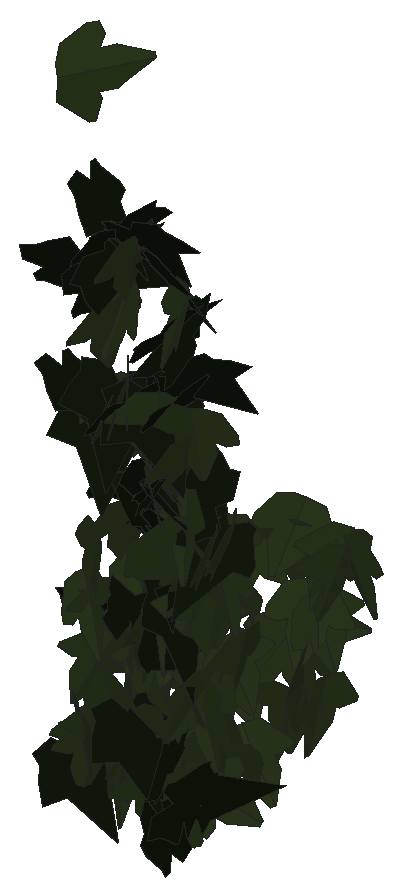
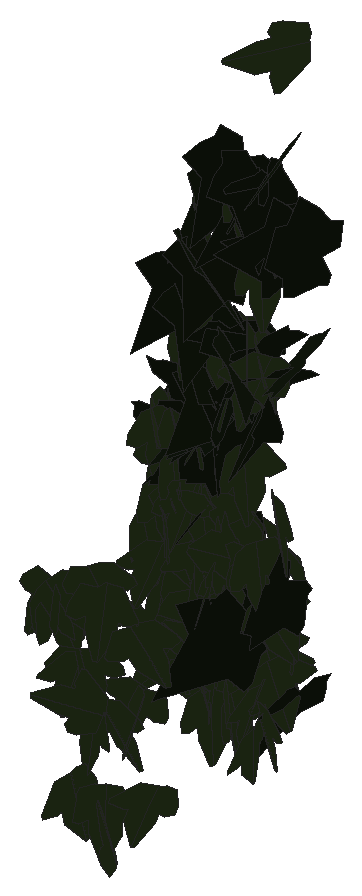
# SketchUp Ruby script. Lengths in inches.
U = 1.inch
M = Sketchup.active_model
def pt(a) = Geom::Point3d.new(a.map { |v| v * U })
def face(e, loops, mat)
  f = e.add_face(loops[0].map { |a| pt(a) })
  loops[1..].each { |l| e.add_face(l.map { |a| pt(a) }).erase! }
  f.material = f.back_material = mat if mat
  f
end
# faces: each face lists its corners as indices into pts; further lists are holes
def faces(e, pts, list, mat = nil) = list.each { |f| face(e, (f[0].is_a?(Array) ? f : [f]).map { |l| l.map { |i| pts[i] } }, mat) }
# xy, xz, yz: faces in a plane at the given z, y or x. An outline is a flat list of corners, or four numbers for a rectangle; further outlines are holes
def ring(l) = l.size == 4 ? [[l[0], l[1]], [l[2], l[1]], [l[2], l[3]], [l[0], l[3]]] : l.each_slice(2).to_a
def flat(e, list, mat, &to3) = list.each { |f| face(e, (f[0].is_a?(Array) ? f : [f]).map { |l| ring(l).map { |u, v| to3.(u, v) } }, mat) }
def xy(e, z, list, mat = nil) = flat(e, list, mat) { |x, y| [x, y, z] }
def xz(e, y, list, mat = nil) = flat(e, list, mat) { |x, z| [x, y, z] }
def yz(e, x, list, mat = nil) = flat(e, list, mat) { |y, z| [x, y, z] }
def lines(e, pts, list) = list.each { |a, b| e.add_line(pt(pts[a]), pt(pts[b])) }
# prism: a flat outline (further loops are holes) pulled along v
def prism(e, loops, v, mat = nil)
  f = face(e, loops, mat); d = Geom::Vector3d.new(v.map { |x| x * U })
  f.pushpull(f.normal.samedirection?(d) ? d.length : -d.length)
end
def box(e, o, s, mat = nil) = prism(e, [[o, [o[0] + s[0], o[1], o[2]], [o[0] + s[0], o[1] + s[1], o[2]], [o[0], o[1] + s[1], o[2]]]], [0, 0, s[2]], mat)
def at(x, y, z, deg = 0) = Geom::Transformation.translation(pt([x, y, z])) * Geom::Transformation.rotation(ORIGIN, Z_AXIS, deg.degrees)
def axes(o, x, y, z) = Geom::Transformation.new([*x, 0, *y, 0, *z, 0, *pt(o).to_a, 1])
def part(name) = M.definitions.add(name)
# library, detail: a bought-in or finely detailed component or shape, given as its bounding box
def library(name, o, s) = part(name).tap { |d| box(d.entities, o, s) }
def detail(e, o, s) = box(e.add_group.entities, o, s)
def put(e, d, t, mat = nil) = e.add_instance(d, t).tap { |i| i.material = mat if mat }
def group(e, t, mat = nil) = e.add_group.tap { |g| g.transformation = t; g.material = mat if mat }.entities
root = M.entities
M.materials.add("efeu1").color = [18, 25, 13]
M.materials.add("efeu2").color = [43, 57, 29]
c1 = part("ivyleaf_10")
p = [[0,0.5,-0.03],[-0.0625,2.02,-0.43],[-0.19,2.01,-0.46],[-0.54,1.05,-0.29],[-0.52,0.625,-0.18],[-0.83,0.76,-0.28],
  [-1.16,0.64,-0.33],[-1.15,0.33,-0.24],[-0.77,-0.39,0.02],[-0.3,-0.51,0.16],[0.04,-0.48,0.23],[-0.02,2.01,-0.4375],
  [-0.06,2.01,-0.43],[0.04,-0.49,0.23],[0.67,-0.49,0.14],[1.38,0.36,-0.2],[1.375,0.51,-0.24],[0.81,0.65,-0.19],
  [0.62,0.59,-0.15],[0.6,1.09,-0.28],[0.5,1.23,-0.31]]
faces(c1.entities,p,[[0,1,2,3,4,5,6,7,8,9,10],[11,12,0,13,14,15,16,17,18,19,20]],"efeu2")
c2 = part("ivyleaf_9")
p = [[1.54,2.16,1.25],[1.36,2.04,1.19],[-0.21,0.99,0.68],[-0.71,1.11,0.82],[-0.85,0.86,0.67],[-0.8,0.17,0.21],
  [-0.9,-0.01,0.1],[-0.67,-0.16,-0.02],[-0.08,-0.08,-0.05],[-0.03,-0.6,-0.4],[0.65,-0.88,-0.66],[0.83,-0.6,-0.49],
  [1.29,-0.42,-0.43],[1.8125,-0.07,-0.26],[1.21,0.44,0.15]]
faces(c2.entities,p,[[0,1,2,3,4,5,6,7,8,9,10,11,12,13,14]],"efeu1")
put(root,c1,axes([532.71,135.74,197.29],[-0.01578,-0.78364,-0.10568],[-0.00617,0.10582,-0.78375],[0.7907,-0.01481,-0.00823]))
put(root,c1,axes([533.85,135.95,191.34],[0.65433,-0.22783,0.34353],[0.31965,-0.12651,-0.69274],[0.26028,0.72812,-0.01287]))
put(root,c2,axes([532.51,135.84,185.99],[0.1547,-0.69949,-0.30265],[-0.0515,0.29852,-0.71627],[0.76041,0.16252,0.01306]))
put(root,c1,axes([532.37,135.86,195.95],[0.68063,-0.39342,-0.05672],[-0.0537,0.02042,-0.7861],[0.39384,0.68268,-0.00917]))
put(root,c1,axes([534.67,135.8,190.9],[0.34135,-0.66357,-0.12192],[-0.06148,0.10547,-0.74619],[0.67187,0.34678,-0.00634]))
put(root,c1,axes([532.12,135.76,195.51],[-0.16929,-0.77066,-0.10479],[0.00055,0.10713,-0.78872],[0.77775,-0.16783,-0.02225]))
put(root,c1,axes([532.18,136.01,185.5],[-0.76316,-0.38571,-0.20662],[-0.16401,-0.13298,0.85399],[-0.40567,0.77938,0.04345]))
put(root,c1,axes([533.82,135.88,196.2],[0.55162,-0.56153,-0.04959],[-0.03593,0.03423,-0.78715],[0.56257,0.55278,-0.00164]))
put(root,c1,axes([531.99,135.89,193.26],[0.3547,-0.68149,-0.01004],[-0.00284,0.00984,-0.76827],[0.68156,0.35471,0.00202]))
put(root,c1,axes([531.58,135.25,201.23],[0.09209,-0.09543,-0.84775],[0.57027,0.64106,-0.01022],[0.63449,-0.56232,0.13222]))
put(root,c2,axes([530.61,135.56,196.14],[0.47102,-0.08261,0.62523],[0.62973,0.10402,-0.46067],[-0.03427,0.77586,0.12833]))
put(root,c2,axes([532.96,135.46,197.81],[0.70238,0.34716,-0.12708],[-0.14154,0.00047,-0.78101],[-0.34152,0.71379,0.06232]))
put(root,c1,axes([531.36,135.7,185.61],[-0.55375,0.44882,0.09771],[-0.10631,0.02367,-0.71117],[-0.44686,-0.5618,0.0481]))
put(root,c2,axes([532.46,135.5,197.67],[0.06107,0.80172,-0.09598],[-0.0084,-0.09562,-0.80404],[-0.8074,0.06163,0.0011]))
put(root,c2,axes([531.93,136.2,193.48],[-0.16369,-0.75491,-0.04148],[0.01357,0.0395,-0.77244],[0.75593,-0.16418,0.00488]))
put(root,c2,axes([531.61,135.78,198.3125],[0.49585,-0.55416,-0.26987],[-0.14219,0.23417,-0.74211],[0.59975,0.51367,0.04717]))
put(root,c2,axes([532.66,135.91,187.8],[-0.31836,0.12735,0.72859],[0.54441,-0.4966,0.32469],[0.50067,0.62096,0.11024]))
put(root,c2,axes([531.66,136.19,192.74],[-0.2289,-0.71927,-0.11469],[0.15314,0.07001,-0.74468],[0.71207,-0.24627,0.12329]))
put(root,c2,axes([533.75,135.62,183.39],[0.03053,-0.07595,0.77658],[-0.46155,0.62487,0.07926],[-0.62913,-0.46211,-0.02046]))
put(root,c1,axes([534.19,136.03,186.89],[0.53208,-0.12201,0.53303],[0.5229,-0.10403,-0.54578],[0.15995,0.74593,0.01107]))
put(root,c2,axes([534.33,135.2,184.83],[0.05794,0.41171,-0.73667],[-0.0236,0.73891,0.4111],[0.84359,-0.0076,0.0621]))
put(root,c1,axes([534.44,136.02,187.3],[0.17122,0.61376,-0.36569],[-0.39727,-0.23076,-0.57331],[-0.59381,0.33136,0.2781]))
put(root,c1,axes([533.88,136.01,183.99],[0.5526,-0.5168,-0.23062],[0.16567,-0.16048,0.75659],[-0.54113,-0.57688,-0.00387]))
put(root,c2,axes([533.9,135.37,185.37],[-0.10285,0.43282,0.64418],[-0.16879,0.62178,-0.44472],[-0.7575,-0.19732,0.01163]))
put(root,c2,axes([532.68,135.66,193.57],[0.03079,0.76078,-0.10846],[-0.03271,-0.10715,-0.76088],[-0.76777,0.03507,0.02807]))
put(root,c2,axes([533.62,135.89,192.31],[-0.48687,0.60868,-0.1465],[0.09945,-0.10804,-0.77938],[-0.61811,-0.49682,-0.01]))
put(root,c1,axes([533.11,136.0625,193.46],[-0.4513,-0.63197,0.06071],[0.0406,-0.10305,-0.77102],[0.63358,-0.44355,0.09265]))
put(root,c1,axes([531.5,136.14,185.125],[-0.22314,-0.68867,0.16461],[-0.0185,-0.16686,-0.72316],[0.70782,-0.22146,0.03299]))
put(root,c2,axes([530.7,135.99,193.51],[0.49485,-0.60004,-0.10096],[0.0412,0.16288,-0.76609],[0.60708,0.47806,0.13429]))
put(root,c1,axes([533.85,135.99,192.79],[-0.01946,-0.77711,-0.08156],[-0.0149,0.08194,-0.77717],[0.78124,-0.0178,-0.01685]))
put(root,c2,axes([533.2,135.73,197.15],[0.76974,-0.06922,-0.18511],[-0.17979,0.06379,-0.77147],[0.08206,0.78911,0.04613]))
put(root,c2,axes([532.26,135.45,197.1],[0.05524,-0.06483,-0.79971],[-0.19864,0.77554,-0.0766],[0.77736,0.20278,0.03725]))
put(root,c2,axes([534.65,136.36,190.98],[-0.66942,-0.3533,-0.10756],[0.10727,0.02707,-0.75648],[0.35339,-0.67746,0.02587]))
put(root,c1,axes([533.97,136.06,190.86],[-0.47931,-0.60258,0.04879],[-0.03165,-0.03716,-0.76996],[0.60372,-0.48035,-0.00163]))
put(root,c1,axes([534.15,136.11,185.64],[-0.83708,0.05836,-0.06664],[-0.06762,-0.01195,0.83895],[0.05722,0.83964,0.01657]))
put(root,c1,axes([533.34,135.8125,190.43],[-0.46319,-0.44413,-0.41452],[0.32715,0.25688,-0.64079],[0.5119,-0.56603,0.03444]))
put(root,c1,axes([531.05,136.1875,188.37],[0.5742,-0.12033,0.47152],[0.46297,-0.0896,-0.58664],[0.14991,0.73757,0.00566]))
put(root,c2,axes([530.86,135.96,184.55],[0.2161,-0.5919,-0.43635],[-0.10081,0.42666,-0.62869],[0.72841,0.23465,0.04245]))
put(root,c2,axes([533.33,136.32,188.77],[0.23023,-0.72264,0.03226],[-0.00802,-0.0364,-0.75819],[0.72331,0.22961,-0.01867]))
put(root,c1,axes([534.13,135.99,193.51],[-0.73996,-0.23205,0.0115],[-0.01098,-0.00343,-0.77549],[0.23208,-0.74004,-0.00001]))
put(root,c2,axes([532.82,136.1,193.59],[-0.10468,-0.60558,-0.46611],[0.14954,0.44514,-0.61191],[0.74942,-0.17341,0.057]))
put(root,c1,axes([533.81,136.35,188.82],[-0.3326,-0.60196,0.33303],[-0.04232,-0.3513,-0.67726],[0.68664,-0.31324,0.11957]))
put(root,c2,axes([533.97,136.04,195.42],[-0.60314,0.49283,0.05882],[-0.04306,0.04025,-0.77887],[-0.49446,-0.60466,-0.00391]))
put(root,c1,axes([534.1,136.05,190.25],[-0.66091,0.33329,0.1311],[-0.18197,-0.07549,-0.72543],[-0.30847,-0.66954,0.14705]))
put(root,c1,axes([533.05,136.11,184.51],[-0.48803,-0.53213,-0.01905],[0.01209,0.01476,-0.72204],[0.53234,-0.48818,-0.00106]))
put(root,c1,axes([532.8,136.21,188.44],[0.17448,-0.72033,-0.01986],[0.00396,0.02139,-0.74111],[0.7206,0.1743,0.00889]))
put(root,c1,axes([532.27,135.98,193.65],[0.28612,-0.64479,-0.33721],[-0.0415,0.34729,-0.69928],[0.72645,0.2738,0.09286]))
put(root,c2,axes([531.5,135.58,195.9],[0.09677,0.15839,0.77598],[0.48866,0.60326,-0.18408],[-0.62326,0.49758,-0.02384]))
put(root,c1,axes([534.75,136.3,190.88],[0.30421,-0.70293,-0.02525],[-0.01678,0.02025,-0.7659],[0.70319,0.30458,-0.00735]))
put(root,c2,axes([534.48,136.125,191.56],[-0.41378,0.26367,0.60094],[-0.53138,0.28226,-0.48972],[-0.38508,-0.67281,0.03005]))
put(root,c2,axes([532.12,136.24,191.11],[0.59286,-0.47398,-0.09523],[-0.085,0.04614,-0.75885],[0.47593,0.59868,-0.01691]))
put(root,c2,axes([532.42,135.9,191.7],[0.4256,0.63773,-0.06908],[-0.0317,-0.06189,-0.76667],[-0.64068,0.42671,-0.00796]))
put(root,c1,axes([532.21,136.36,189.14],[0.57111,-0.00047,0.50179],[0.50176,0.00897,-0.57106],[-0.00557,0.76018,0.00705]))
put(root,c1,axes([531.24,136.24,189.43],[0.54798,-0.47906,-0.21151],[-0.08203,0.22384,-0.7195],[0.51721,0.54306,0.10998]))
put(root,c1,axes([531.18,136.52,185.13],[-0.25826,-0.6733,0.21834],[0.01197,-0.23654,-0.71527],[0.70772,-0.2417,0.09178]))
put(root,c1,axes([533.84,136.76,187.02],[-0.06332,-0.50996,0.52438],[0.18919,-0.51985,-0.4827],[0.70657,0.0935,0.17624]))
put(root,c2,axes([533.01,136.13,190.47],[0.73125,-0.04405,0.22609],[0.22488,-0.02636,-0.73247],[0.04985,0.76495,-0.01222]))
put(root,c2,axes([533.08,136.1,191.35],[0.7224,-0.24136,-0.08905],[-0.02659,0.19399,-0.74143],[0.25589,0.70154,0.17438]))
put(root,c1,axes([532.07,136.4,190.53],[-0.19369,-0.73387,-0.05112],[0.02316,0.04676,-0.75893],[0.73529,-0.19479,0.01044]))
put(root,c1,axes([532.9,136.13,191.57],[-0.44172,0.56271,0.28584],[-0.21938,0.19025,-0.71355],[-0.5918,-0.49054,0.05116]))
put(root,c1,axes([531.25,136.6875,186.85],[-0.28102,-0.56579,0.36102],[-0.12291,-0.34139,-0.6307],[0.65981,-0.30457,0.03628]))
put(root,c2,axes([533.72,135.91,193.87],[0.14506,0.74057,0.18573],[-0.02466,0.1935,-0.75229],[-0.76311,0.13452,0.05962]))
put(root,c2,axes([532.77,136.31,191.87],[0.70312,-0.27942,-0.14049],[-0.12887,0.05612,-0.75659],[0.28497,0.71482,0.00449]))
put(root,c2,axes([533.9,135.99,194.56],[0.61298,0.46137,0.1288],[0.1087,0.06974,-0.76715],[-0.46651,0.62247,-0.00951]))
put(root,c1,axes([532.45,136.61,187.93],[0.03735,-0.72589,0.08729],[0.01411,-0.08667,-0.72679],[0.73098,0.03876,0.00957]))
put(root,c1,axes([534.38,136.49,190.78],[-0.54377,-0.52106,-0.05839],[0.11609,-0.03761,-0.74546],[0.51131,-0.5456,0.10715]))
put(root,c1,axes([532.21,136.42,188.94],[0.43521,0.14891,0.60494],[0.58236,0.16491,-0.45955],[-0.22132,0.72675,-0.01967]))
put(root,c1,axes([534.27,136.56,189.03],[-0.39733,-0.6152,0.06936],[-0.02119,-0.06885,-0.73209],[0.61873,-0.39742,0.01947]))
put(root,c1,axes([533.37,136.49,189.31],[-0.64561,-0.33849,0.13887],[-0.12819,-0.05453,-0.72887],[0.34267,-0.65812,-0.01103]))
put(root,c1,axes([533.26,136.65,187.61],[0.42001,-0.59435,-0.01457],[-0.02155,0.00261,-0.7276],[0.59414,0.42026,-0.01609]))
put(root,c1,axes([534.39,136.6,189.87],[-0.68988,0.22,-0.17958],[0.12106,-0.19893,-0.70877],[-0.25689,-0.68455,0.14826]))
put(root,c1,axes([531.63,136.25,193.03],[0.339,0.60122,0.3422],[0.01569,0.3743,-0.67316],[-0.6916,0.30319,0.15246]))
put(root,c1,axes([532.67,136.74,187.27],[-0.38651,-0.59117,0.1928],[-0.02961,-0.20926,-0.70098],[0.62111,-0.37785,0.08656]))
put(root,c2,axes([533.28,136.01,195.28],[0.22556,0.70831,0.24547],[0.00301,0.25549,-0.73997],[-0.74964,0.21415,0.07089]))
put(root,c1,axes([533.94,136.64,189.88],[-0.01379,-0.7478,-0.01243],[-0.00341,0.01249,-0.74792],[0.74789,-0.01373,-0.00364]))
put(root,c1,axes([531.46,136.7,188.28],[-0.28787,-0.68469,0.04176],[0.01909,-0.05327,-0.74176],[0.68569,-0.28597,0.03819]))
put(root,c1,axes([532.41,136.875,187.89],[-0.44674,-0.49018,0.31632],[-0.10061,-0.32771,-0.64992],[0.57464,-0.43845,0.13212]))
put(root,c1,axes([534.7,136.82,188.07],[-0.00148,-0.7324,0.05146],[0.01947,-0.05148,-0.73215],[0.73395,-0.00011,0.01952]))
put(root,c2,axes([533.07,136.11,191.67],[0.30286,0.53285,0.46477],[0.11362,0.46237,-0.60413],[-0.69788,0.30652,0.10334]))
put(root,c1,axes([534.2,136.3,184.62],[0.14167,0.4354,0.58589],[0.19341,0.5531,-0.45781],[-0.70387,0.23962,-0.00787]))
put(root,c1,axes([532.27,136.71,187.94],[-0.70557,-0.19777,0.04434],[-0.04233,-0.01329,-0.73276],[0.19821,-0.70684,0.00137]))
put(root,c1,axes([531.93,136.74,185.98],[-0.20813,0.68277,-0.11379],[0.0298,-0.10987,-0.71378],[-0.69155,-0.21022,0.00349]))
put(root,c1,axes([533.68,136.79,189.07],[0.69899,0.21357,0.00506],[-0.00846,0.04498,-0.72947],[-0.21346,0.69756,0.04549]))
put(root,c1,axes([532.85,136.5,184.76],[-0.31118,0.56364,0.32562],[-0.26224,0.22178,-0.6345],[-0.59578,-0.39201,0.10922]))
put(root,c1,axes([533.04,136.89,188.03],[0.50126,0.49042,-0.18621],[-0.13901,-0.12416,-0.70122],[-0.50583,0.52011,0.00818]))
put(root,c1,axes([533.48,136.66,189.18],[-0.44863,-0.5329,-0.27498],[0.20618,0.18541,-0.69569],[0.5631,-0.49246,0.03565]))
put(root,c1,axes([533.05,136.98,185.62],[0.59505,-0.3705,0.19471],[0.18065,-0.07794,-0.7004],[0.37755,0.62122,0.02825]))
put(root,c1,axes([534.36,136.94,185.14],[-0.87986,0.00114,-0.04807],[-0.04808,-0.024,0.87953],[-0.00018,0.88085,0.02402]))
put(root,c2,axes([532.33,136.34,193.02],[-0.137,0.55474,0.51307],[-0.18252,0.4817,-0.56956],[-0.73325,-0.22355,0.04591]))
put(root,c2,axes([530.79,136.54,187.77],[0.82738,0.13468,-0.12334],[-0.12247,-0.01528,-0.83826],[-0.13547,0.83639,0.00454]))
put(root,c1,axes([531.2,136.89,184.32],[0.57474,-0.40155,-0.1105],[-0.07471,0.08585,-0.70059],[0.40972,0.57894,0.02724]))
put(root,c1,axes([533,137.05,184.47],[0.37771,-0.25759,-0.56297],[0.46597,-0.31593,0.45718],[-0.40763,-0.59982,0.00097]))
put(root,c1,axes([532.48,136.87,185.18],[0.61657,0.36267,0.07531],[0.0501,0.06324,-0.71474],[-0.367,0.61793,0.02895]))
put(root,c1,axes([532.83,136.98,187.59],[0.38708,-0.60528,-0.07917],[-0.03609,0.07089,-0.71843],[0.60937,0.38868,0.00774]))
put(root,c1,axes([533.59,137.34,186.24],[0.14819,0.35248,-0.60973],[-0.43204,-0.44657,-0.36316],[-0.5562,0.4408,0.11964]))
put(root,c1,axes([532.24,136.96,186.63],[-0.68806,-0.1788,0.09769],[-0.09829,-0.01011,-0.71076],[0.17848,-0.69489,-0.0148]))
put(root,c1,axes([532.57,137.0625,184.16],[-0.34402,-0.6289,-0.01701],[0.00919,0.01436,-0.71684],[0.62906,-0.34415,0.00117]))
put(root,c1,axes([531.72,137.2,184.39],[0.0453,-0.71444,-0.00629],[-0.02118,0.00496,-0.71557],[0.71416,0.04547,-0.02082]))
put(root,c1,axes([532.39,136.65,187.92],[0.10475,-0.48607,0.70488],[-0.18613,0.68022,0.49673],[-0.83575,-0.21242,-0.02228]))
put(root,c1,axes([534.01,136.95,188.13],[0.4874,-0.3415,0.42417],[-0.34133,0.25196,0.59507],[-0.42431,-0.59498,0.00854]))
put(root,c1,axes([531.31,137.03,184.81],[-0.13431,0.69408,0.08027],[-0.01393,0.07906,-0.70696],[-0.69857,-0.13503,-0.00134]))
put(root,c1,axes([532.48,136.8,187.51],[0.05311,-0.44146,-0.5868],[0.05603,0.58906,-0.43809],[0.73218,-0.01306,0.07609]))
put(root,c1,axes([534.25,136.97,187.55],[0.19431,0.65773,0.24751],[0.03301,0.24797,-0.68487],[-0.70198,0.19372,0.03631]))
put(root,c1,axes([531.83,137.25,184.73],[0.24141,-0.6636,-0.10336],[0.00882,0.11295,-0.70462],[0.67154,0.23707,0.04641]))
put(root,c1,axes([532.69,137.07,185.29],[-0.35859,-0.33781,0.53088],[0.38532,0.36519,0.49265],[-0.49748,0.52636,-0.00109]))
put(root,c1,axes([532.74,137.37,185.49],[0.36437,-0.6172,-0.02093],[-0.00951,0.01869,-0.71672],[0.61748,0.36449,0.00131]))
put(root,c1,axes([531.17,137.32,183.85],[-0.09715,0.68383,-0.15728],[-0.05351,-0.16553,-0.68668],[-0.69964,-0.08229,0.07436]))
put(root,c2,axes([531.47,137.51,186.59],[0.63519,0.4711,0.32823],[0.26172,0.1981,-0.79082],[-0.51105,0.68699,0.00296]))
put(root,c1,axes([533.5625,138.43,184.63],[0.56342,0.284,0.34909],[0.30969,0.16115,-0.63093],[-0.32651,0.64291,0.00394]))
put(root,c1,axes([534.91,138.3125,186.22],[-0.04606,0.19606,0.70271],[-0.4823,0.52011,-0.17672],[-0.54738,-0.47477,0.09658]))
put(root,c1,axes([533.17,140.625,188.93],[0.6447,0.2788,-0.20265],[-0.19547,-0.05828,-0.70201],[-0.28388,0.67328,0.02314]))
put(root,c1,axes([531.9,140.61,187.74],[0.57995,0.31896,-0.30182],[-0.31209,-0.05235,-0.655],[-0.30891,0.65169,0.09511]))
put(root,c1,axes([534.01,140.98,188.01],[-0.18208,-0.6642,0.23474],[-0.0074,-0.24064,-0.68663],[0.70442,-0.17421,0.05346]))
put(root,c1,axes([534.03,141.08,188.34],[-0.28239,-0.59066,0.38104],[-0.0207,-0.40348,-0.64078],[0.7026,-0.24929,0.13427]))
put(root,c1,axes([532.9,140.68,188.43],[-0.73004,-0.1153,0.03776],[-0.03847,0.00156,-0.73905],[0.11507,-0.73101,-0.00754]))
put(root,c1,axes([533.26,140.91,186.82],[0.6916,0.28041,-0.0603],[-0.05593,-0.02255,-0.74628],[-0.28132,0.69385,0.00012]))
put(root,c1,axes([532.51,140.87,185.61],[0.63291,-0.18161,-0.33964],[-0.32478,0.09952,-0.65843],[0.20702,0.71136,0.0054]))
put(root,c1,axes([534.32,141.02,188.29],[-0.61361,0.29379,-0.26503],[0.21159,-0.16962,-0.67789],[-0.33434,-0.64652,0.05741]))
put(root,c1,axes([531.67,140.94,186.08],[-0.41422,0.57906,-0.04144],[0.0302,-0.02934,-0.71192],[-0.57976,-0.41525,-0.00747]))
put(root,c1,axes([533.46,140.9,186.625],[0.21873,0.67018,0.1664],[0.01397,0.17022,-0.70392],[-0.69039,0.21577,0.03848]))
put(root,c1,axes([532.8,141.21,185.54],[-0.66615,0.26235,0.00767],[-0.04226,-0.08656,-0.70948],[-0.25903,-0.66054,0.09602]))
put(root,c1,axes([530.86,141.37,184.19],[0.34112,0.57335,0.2312],[0.09077,0.21475,-0.66647],[-0.61151,0.3517,0.03005]))
put(root,c1,axes([532.72,141.35,185.83],[-0.09596,-0.02984,0.71109],[0.60198,0.37938,0.09716],[-0.37968,0.60904,-0.02568]))
put(root,c1,axes([532.12,141.63,183.75],[-0.70545,-0.1772,0.10149],[-0.0953,-0.03717,-0.72726],[0.18061,-0.71175,0.01271]))
put(root,c1,axes([531.79,141.79,182.57],[0.42529,-0.58283,0.08136],[-0.05895,0.05769,0.72137],[-0.58552,-0.42914,-0.01353]))
put(root,c1,axes([532.86,141.87,184.01],[0.07422,0.72377,-0.09823],[-0.27044,-0.06449,-0.67949],[-0.67849,0.10487,0.26009]))
